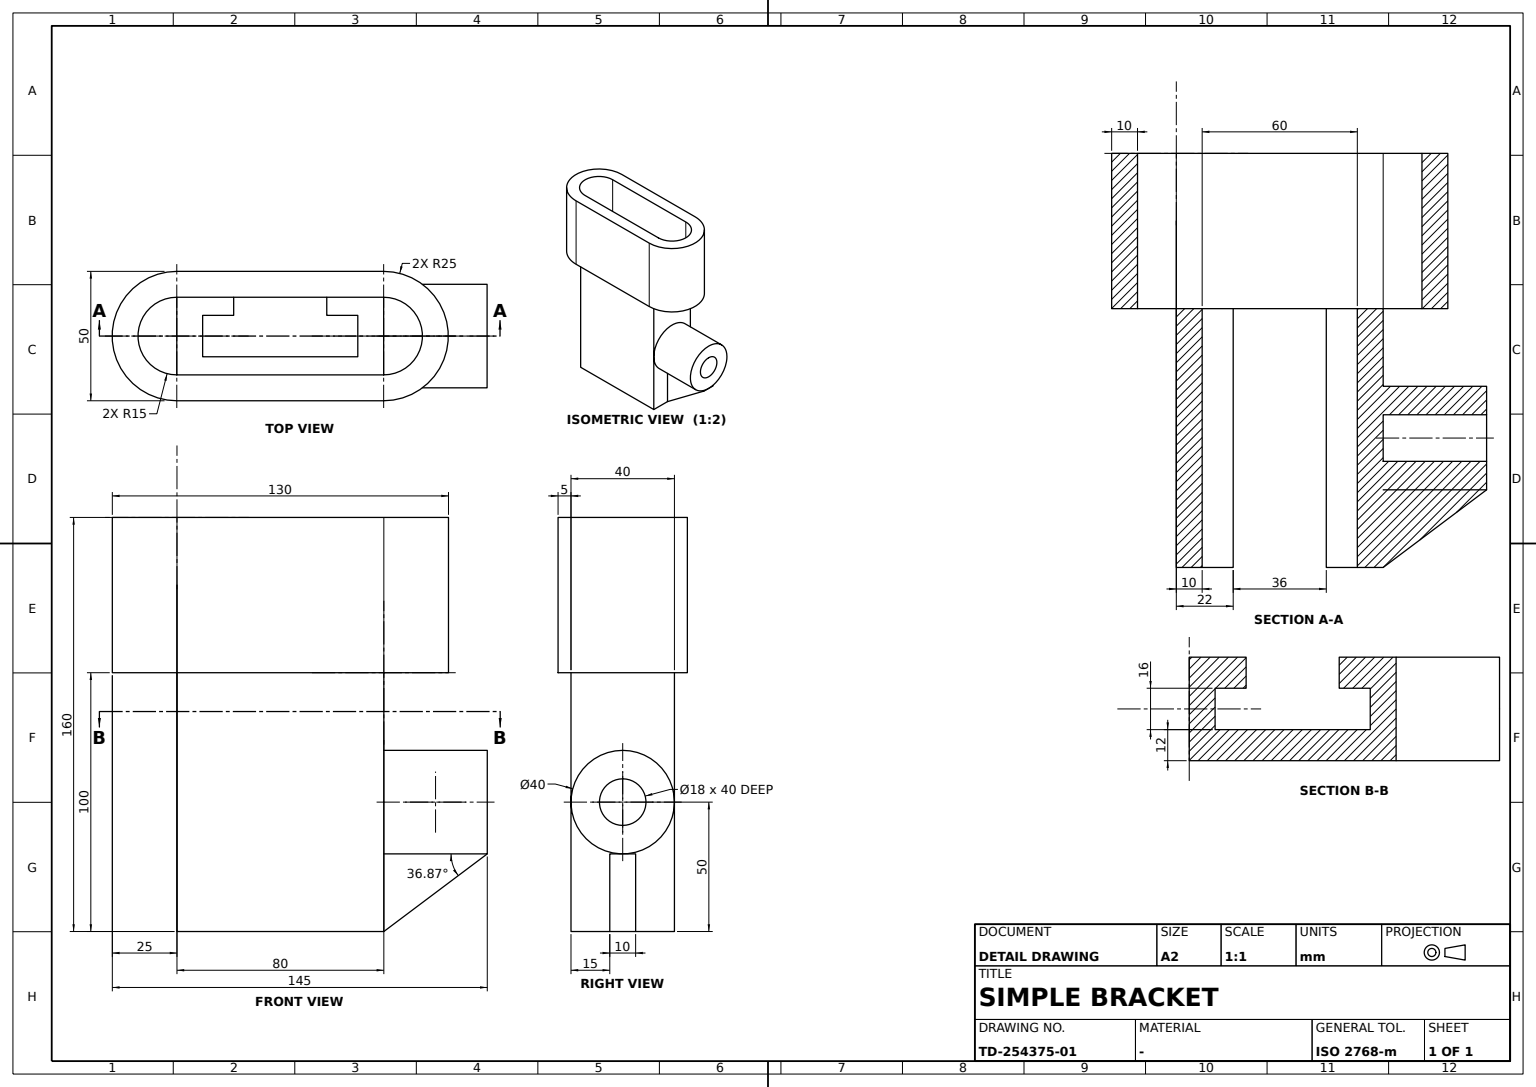
ISO-10303-21;
HEADER;
FILE_DESCRIPTION((''),'2;1');
FILE_NAME('','',(''),(''),'','','');
FILE_SCHEMA(('AUTOMOTIVE_DESIGN'));
ENDSEC;
DATA;
#1=APPLICATION_CONTEXT('');
#2=PRODUCT_CONTEXT('',#1,'mechanical');
#3=PRODUCT('','','',(#2));
#4=PRODUCT_DEFINITION_FORMATION('','',#3);
#5=PRODUCT_DEFINITION_CONTEXT('',#1,'design');
#6=PRODUCT_DEFINITION('','',#4,#5);
#7=PRODUCT_DEFINITION_SHAPE('','',#6);
#8=(LENGTH_UNIT()NAMED_UNIT(*)SI_UNIT(.MILLI.,.METRE.));
#9=(NAMED_UNIT(*)PLANE_ANGLE_UNIT()SI_UNIT($,.RADIAN.));
#10=(NAMED_UNIT(*)SI_UNIT($,.STERADIAN.)SOLID_ANGLE_UNIT());
#11=UNCERTAINTY_MEASURE_WITH_UNIT(LENGTH_MEASURE(0.005),#8,'distance_accuracy_value','');
#12=(GEOMETRIC_REPRESENTATION_CONTEXT(3)GLOBAL_UNCERTAINTY_ASSIGNED_CONTEXT((#11))GLOBAL_UNIT_ASSIGNED_CONTEXT((#8,#9,#10))REPRESENTATION_CONTEXT('',''));
#13=CARTESIAN_POINT('',(-15.,-58.,100.));
#14=VERTEX_POINT('',#13);
#15=CARTESIAN_POINT('',(-15.,-80.,100.));
#16=VERTEX_POINT('',#15);
#17=CARTESIAN_POINT('',(-15.,0.,100.));
#18=DIRECTION('',(0.,-1.,0.));
#19=VECTOR('',#18,1000.);
#20=LINE('',#17,#19);
#21=EDGE_CURVE('',#14,#16,#20,.T.);
#22=ORIENTED_EDGE('',*,*,#21,.F.);
#23=CARTESIAN_POINT('',(-15.,-22.,100.));
#24=VERTEX_POINT('',#23);
#25=EDGE_CURVE('',#24,#14,#20,.T.);
#26=ORIENTED_EDGE('',*,*,#25,.F.);
#27=VERTEX_POINT('',#17);
#28=EDGE_CURVE('',#27,#24,#20,.T.);
#29=ORIENTED_EDGE('',*,*,#28,.F.);
#30=CARTESIAN_POINT('',(-15.,0.,160.));
#31=VERTEX_POINT('',#30);
#32=CARTESIAN_POINT('',(-15.,0.,130.));
#33=DIRECTION('',(0.,0.,1.));
#34=VECTOR('',#33,1000.);
#35=LINE('',#32,#34);
#36=EDGE_CURVE('',#27,#31,#35,.T.);
#37=ORIENTED_EDGE('',*,*,#36,.T.);
#38=CARTESIAN_POINT('',(-15.,-80.,160.));
#39=VERTEX_POINT('',#38);
#40=LINE('',#30,#19);
#41=EDGE_CURVE('',#31,#39,#40,.T.);
#42=ORIENTED_EDGE('',*,*,#41,.T.);
#43=CARTESIAN_POINT('',(-15.,-80.,130.));
#44=LINE('',#43,#34);
#45=EDGE_CURVE('',#16,#39,#44,.T.);
#46=ORIENTED_EDGE('',*,*,#45,.F.);
#47=EDGE_LOOP('',(#22,#26,#29,#37,#42,#46));
#48=FACE_BOUND('',#47,.T.);
#49=DIRECTION('',(-1.,0.,0.));
#50=AXIS2_PLACEMENT_3D('',#17,#49,#18);
#51=PLANE('',#50);
#52=ADVANCED_FACE('',(#48),#51,.F.);
#53=CARTESIAN_POINT('',(15.,-80.,160.));
#54=VERTEX_POINT('',#53);
#55=CARTESIAN_POINT('',(0.,-80.,160.));
#56=DIRECTION('',(1.,0.,0.));
#57=AXIS2_PLACEMENT_3D('',#55,#33,#56);
#58=CIRCLE('',#57,15.);
#59=EDGE_CURVE('',#39,#54,#58,.T.);
#60=ORIENTED_EDGE('',*,*,#59,.T.);
#61=CARTESIAN_POINT('',(15.,-80.,100.));
#62=VERTEX_POINT('',#61);
#63=CARTESIAN_POINT('',(15.,-80.,130.));
#64=LINE('',#63,#34);
#65=EDGE_CURVE('',#62,#54,#64,.T.);
#66=ORIENTED_EDGE('',*,*,#65,.F.);
#67=CARTESIAN_POINT('',(0.,-80.,100.));
#68=AXIS2_PLACEMENT_3D('',#67,#33,#56);
#69=CIRCLE('',#68,15.);
#70=EDGE_CURVE('',#16,#62,#69,.T.);
#71=ORIENTED_EDGE('',*,*,#70,.F.);
#72=ORIENTED_EDGE('',*,*,#45,.T.);
#73=EDGE_LOOP('',(#60,#66,#71,#72));
#74=FACE_BOUND('',#73,.T.);
#75=CARTESIAN_POINT('',(0.,-80.,130.));
#76=AXIS2_PLACEMENT_3D('',#75,#33,#56);
#77=CYLINDRICAL_SURFACE('',#76,15.);
#78=ADVANCED_FACE('',(#74),#77,.F.);
#79=CARTESIAN_POINT('',(-8.,-58.,0.));
#80=VERTEX_POINT('',#79);
#81=CARTESIAN_POINT('',(-8.,-70.,0.));
#82=VERTEX_POINT('',#81);
#83=CARTESIAN_POINT('',(-8.,0.,0.));
#84=LINE('',#83,#19);
#85=EDGE_CURVE('',#80,#82,#84,.T.);
#86=ORIENTED_EDGE('',*,*,#85,.F.);
#87=CARTESIAN_POINT('',(-8.,-58.,100.));
#88=VERTEX_POINT('',#87);
#89=LINE('',#79,#34);
#90=EDGE_CURVE('',#80,#88,#89,.T.);
#91=ORIENTED_EDGE('',*,*,#90,.T.);
#92=CARTESIAN_POINT('',(-8.,-70.,100.));
#93=VERTEX_POINT('',#92);
#94=CARTESIAN_POINT('',(-8.,0.,100.));
#95=LINE('',#94,#19);
#96=EDGE_CURVE('',#88,#93,#95,.T.);
#97=ORIENTED_EDGE('',*,*,#96,.T.);
#98=LINE('',#81,#34);
#99=EDGE_CURVE('',#82,#93,#98,.T.);
#100=ORIENTED_EDGE('',*,*,#99,.F.);
#101=EDGE_LOOP('',(#86,#91,#97,#100));
#102=FACE_BOUND('',#101,.T.);
#103=CARTESIAN_POINT('',(-8.,-10.,0.));
#104=AXIS2_PLACEMENT_3D('',#103,#49,#18);
#105=PLANE('',#104);
#106=ADVANCED_FACE('',(#102),#105,.F.);
#107=CARTESIAN_POINT('',(-20.,-58.,0.));
#108=VERTEX_POINT('',#107);
#109=CARTESIAN_POINT('',(0.,-58.,0.));
#110=VECTOR('',#56,1000.);
#111=LINE('',#109,#110);
#112=EDGE_CURVE('',#108,#80,#111,.T.);
#113=ORIENTED_EDGE('',*,*,#112,.F.);
#114=CARTESIAN_POINT('',(-20.,-58.,100.));
#115=VERTEX_POINT('',#114);
#116=LINE('',#107,#34);
#117=EDGE_CURVE('',#108,#115,#116,.T.);
#118=ORIENTED_EDGE('',*,*,#117,.T.);
#119=CARTESIAN_POINT('',(0.,-58.,100.));
#120=LINE('',#119,#110);
#121=EDGE_CURVE('',#115,#14,#120,.T.);
#122=ORIENTED_EDGE('',*,*,#121,.T.);
#123=EDGE_CURVE('',#14,#88,#120,.T.);
#124=ORIENTED_EDGE('',*,*,#123,.T.);
#125=ORIENTED_EDGE('',*,*,#90,.F.);
#126=EDGE_LOOP('',(#113,#118,#122,#124,#125));
#127=FACE_BOUND('',#126,.T.);
#128=AXIS2_PLACEMENT_3D('',#107,#18,#56);
#129=PLANE('',#128);
#130=ADVANCED_FACE('',(#127),#129,.F.);
#131=CARTESIAN_POINT('',(-5.,0.,0.));
#132=VERTEX_POINT('',#131);
#133=CARTESIAN_POINT('',(-5.,40.,30.));
#134=VERTEX_POINT('',#133);
#135=DIRECTION('',(0.,0.8,0.6));
#136=VECTOR('',#135,1000.);
#137=LINE('',#131,#136);
#138=EDGE_CURVE('',#132,#134,#137,.T.);
#139=ORIENTED_EDGE('',*,*,#138,.F.);
#140=CARTESIAN_POINT('',(-5.,0.,30.));
#141=VERTEX_POINT('',#140);
#142=DIRECTION('',(0.,0.,-1.));
#143=VECTOR('',#142,1000.);
#144=LINE('',#131,#143);
#145=EDGE_CURVE('',#141,#132,#144,.T.);
#146=ORIENTED_EDGE('',*,*,#145,.F.);
#147=LINE('',#140,#19);
#148=EDGE_CURVE('',#134,#141,#147,.T.);
#149=ORIENTED_EDGE('',*,*,#148,.F.);
#150=EDGE_LOOP('',(#139,#146,#149));
#151=FACE_BOUND('',#150,.T.);
#152=DIRECTION('',(0.,1.,0.));
#153=AXIS2_PLACEMENT_3D('',#131,#56,#152);
#154=PLANE('',#153);
#155=ADVANCED_FACE('',(#151),#154,.F.);
#156=ORIENTED_EDGE('',*,*,#148,.T.);
#157=CARTESIAN_POINT('',(0.,0.,30.));
#158=VERTEX_POINT('',#157);
#159=LINE('',#157,#110);
#160=EDGE_CURVE('',#141,#158,#159,.T.);
#161=ORIENTED_EDGE('',*,*,#160,.T.);
#162=CARTESIAN_POINT('',(5.,0.,30.));
#163=VERTEX_POINT('',#162);
#164=EDGE_CURVE('',#158,#163,#159,.T.);
#165=ORIENTED_EDGE('',*,*,#164,.T.);
#166=CARTESIAN_POINT('',(5.,40.,30.));
#167=VERTEX_POINT('',#166);
#168=LINE('',#162,#19);
#169=EDGE_CURVE('',#167,#163,#168,.T.);
#170=ORIENTED_EDGE('',*,*,#169,.F.);
#171=CARTESIAN_POINT('',(0.,40.,30.));
#172=LINE('',#171,#110);
#173=EDGE_CURVE('',#134,#167,#172,.T.);
#174=ORIENTED_EDGE('',*,*,#173,.F.);
#175=EDGE_LOOP('',(#156,#161,#165,#170,#174));
#176=FACE_BOUND('',#175,.T.);
#177=AXIS2_PLACEMENT_3D('',#171,#33,#18);
#178=PLANE('',#177);
#179=ADVANCED_FACE('',(#176),#178,.T.);
#180=CARTESIAN_POINT('',(-8.,-22.,100.));
#181=VERTEX_POINT('',#180);
#182=CARTESIAN_POINT('',(0.,-22.,100.));
#183=VECTOR('',#49,1000.);
#184=LINE('',#182,#183);
#185=EDGE_CURVE('',#181,#24,#184,.T.);
#186=ORIENTED_EDGE('',*,*,#185,.T.);
#187=CARTESIAN_POINT('',(-20.,-22.,100.));
#188=VERTEX_POINT('',#187);
#189=EDGE_CURVE('',#24,#188,#184,.T.);
#190=ORIENTED_EDGE('',*,*,#189,.T.);
#191=CARTESIAN_POINT('',(-20.,-22.,0.));
#192=VERTEX_POINT('',#191);
#193=LINE('',#191,#34);
#194=EDGE_CURVE('',#192,#188,#193,.T.);
#195=ORIENTED_EDGE('',*,*,#194,.F.);
#196=CARTESIAN_POINT('',(-8.,-22.,0.));
#197=VERTEX_POINT('',#196);
#198=CARTESIAN_POINT('',(0.,-22.,0.));
#199=LINE('',#198,#183);
#200=EDGE_CURVE('',#197,#192,#199,.T.);
#201=ORIENTED_EDGE('',*,*,#200,.F.);
#202=LINE('',#196,#34);
#203=EDGE_CURVE('',#197,#181,#202,.T.);
#204=ORIENTED_EDGE('',*,*,#203,.T.);
#205=EDGE_LOOP('',(#186,#190,#195,#201,#204));
#206=FACE_BOUND('',#205,.T.);
#207=AXIS2_PLACEMENT_3D('',#196,#152,#49);
#208=PLANE('',#207);
#209=ADVANCED_FACE('',(#206),#208,.F.);
#210=ORIENTED_EDGE('',*,*,#203,.F.);
#211=VERTEX_POINT('',#103);
#212=EDGE_CURVE('',#211,#197,#84,.T.);
#213=ORIENTED_EDGE('',*,*,#212,.F.);
#214=CARTESIAN_POINT('',(-8.,-10.,100.));
#215=VERTEX_POINT('',#214);
#216=LINE('',#103,#34);
#217=EDGE_CURVE('',#211,#215,#216,.T.);
#218=ORIENTED_EDGE('',*,*,#217,.T.);
#219=EDGE_CURVE('',#215,#181,#95,.T.);
#220=ORIENTED_EDGE('',*,*,#219,.T.);
#221=EDGE_LOOP('',(#210,#213,#218,#220));
#222=FACE_BOUND('',#221,.T.);
#223=ADVANCED_FACE('',(#222),#105,.F.);
#224=ORIENTED_EDGE('',*,*,#112,.T.);
#225=ORIENTED_EDGE('',*,*,#85,.T.);
#226=CARTESIAN_POINT('',(8.,-70.,0.));
#227=VERTEX_POINT('',#226);
#228=CARTESIAN_POINT('',(0.,-70.,0.));
#229=LINE('',#228,#110);
#230=EDGE_CURVE('',#82,#227,#229,.T.);
#231=ORIENTED_EDGE('',*,*,#230,.T.);
#232=CARTESIAN_POINT('',(8.,-10.,0.));
#233=VERTEX_POINT('',#232);
#234=CARTESIAN_POINT('',(8.,0.,0.));
#235=VECTOR('',#152,1000.);
#236=LINE('',#234,#235);
#237=EDGE_CURVE('',#227,#233,#236,.T.);
#238=ORIENTED_EDGE('',*,*,#237,.T.);
#239=CARTESIAN_POINT('',(0.,-10.,0.));
#240=LINE('',#239,#183);
#241=EDGE_CURVE('',#233,#211,#240,.T.);
#242=ORIENTED_EDGE('',*,*,#241,.T.);
#243=ORIENTED_EDGE('',*,*,#212,.T.);
#244=ORIENTED_EDGE('',*,*,#200,.T.);
#245=CARTESIAN_POINT('',(-20.,0.,0.));
#246=VERTEX_POINT('',#245);
#247=LINE('',#245,#235);
#248=EDGE_CURVE('',#192,#246,#247,.T.);
#249=ORIENTED_EDGE('',*,*,#248,.T.);
#250=CARTESIAN_POINT('',(0.,0.,0.));
#251=LINE('',#250,#110);
#252=EDGE_CURVE('',#246,#132,#251,.T.);
#253=ORIENTED_EDGE('',*,*,#252,.T.);
#254=CARTESIAN_POINT('',(5.,0.,0.));
#255=VERTEX_POINT('',#254);
#256=EDGE_CURVE('',#132,#255,#251,.T.);
#257=ORIENTED_EDGE('',*,*,#256,.T.);
#258=CARTESIAN_POINT('',(20.,0.,0.));
#259=VERTEX_POINT('',#258);
#260=EDGE_CURVE('',#255,#259,#251,.T.);
#261=ORIENTED_EDGE('',*,*,#260,.T.);
#262=CARTESIAN_POINT('',(20.,-80.,0.));
#263=VERTEX_POINT('',#262);
#264=LINE('',#258,#19);
#265=EDGE_CURVE('',#259,#263,#264,.T.);
#266=ORIENTED_EDGE('',*,*,#265,.T.);
#267=CARTESIAN_POINT('',(-20.,-80.,0.));
#268=VERTEX_POINT('',#267);
#269=CARTESIAN_POINT('',(0.,-80.,0.));
#270=LINE('',#269,#183);
#271=EDGE_CURVE('',#263,#268,#270,.T.);
#272=ORIENTED_EDGE('',*,*,#271,.T.);
#273=EDGE_CURVE('',#268,#108,#247,.T.);
#274=ORIENTED_EDGE('',*,*,#273,.T.);
#275=EDGE_LOOP('',(#224,#225,#231,#238,#242,#243,#244,#249,#253,#257,#261,#266,#272,#274));
#276=FACE_BOUND('',#275,.T.);
#277=AXIS2_PLACEMENT_3D('',#250,#33,#56);
#278=PLANE('',#277);
#279=ADVANCED_FACE('',(#276),#278,.F.);
#280=ORIENTED_EDGE('',*,*,#194,.T.);
#281=CARTESIAN_POINT('',(-20.,0.,100.));
#282=VERTEX_POINT('',#281);
#283=LINE('',#281,#235);
#284=EDGE_CURVE('',#188,#282,#283,.T.);
#285=ORIENTED_EDGE('',*,*,#284,.T.);
#286=CARTESIAN_POINT('',(-20.,0.,50.));
#287=VERTEX_POINT('',#286);
#288=LINE('',#245,#34);
#289=EDGE_CURVE('',#287,#282,#288,.T.);
#290=ORIENTED_EDGE('',*,*,#289,.F.);
#291=EDGE_CURVE('',#246,#287,#288,.T.);
#292=ORIENTED_EDGE('',*,*,#291,.F.);
#293=ORIENTED_EDGE('',*,*,#248,.F.);
#294=EDGE_LOOP('',(#280,#285,#290,#292,#293));
#295=FACE_BOUND('',#294,.T.);
#296=AXIS2_PLACEMENT_3D('',#191,#56,#152);
#297=PLANE('',#296);
#298=ADVANCED_FACE('',(#295),#297,.F.);
#299=CARTESIAN_POINT('',(25.,0.,100.));
#300=VERTEX_POINT('',#299);
#301=CARTESIAN_POINT('',(-25.,0.,100.));
#302=VERTEX_POINT('',#301);
#303=CARTESIAN_POINT('',(0.,0.,100.));
#304=AXIS2_PLACEMENT_3D('',#303,#33,#56);
#305=CIRCLE('',#304,25.);
#306=EDGE_CURVE('',#300,#302,#305,.T.);
#307=ORIENTED_EDGE('',*,*,#306,.T.);
#308=CARTESIAN_POINT('',(-25.,0.,160.));
#309=VERTEX_POINT('',#308);
#310=CARTESIAN_POINT('',(-25.,0.,130.));
#311=LINE('',#310,#34);
#312=EDGE_CURVE('',#302,#309,#311,.T.);
#313=ORIENTED_EDGE('',*,*,#312,.T.);
#314=CARTESIAN_POINT('',(25.,0.,160.));
#315=VERTEX_POINT('',#314);
#316=CARTESIAN_POINT('',(0.,0.,160.));
#317=AXIS2_PLACEMENT_3D('',#316,#33,#56);
#318=CIRCLE('',#317,25.);
#319=EDGE_CURVE('',#315,#309,#318,.T.);
#320=ORIENTED_EDGE('',*,*,#319,.F.);
#321=CARTESIAN_POINT('',(25.,0.,130.));
#322=LINE('',#321,#34);
#323=EDGE_CURVE('',#300,#315,#322,.T.);
#324=ORIENTED_EDGE('',*,*,#323,.F.);
#325=EDGE_LOOP('',(#307,#313,#320,#324));
#326=FACE_BOUND('',#325,.T.);
#327=CARTESIAN_POINT('',(0.,0.,130.));
#328=AXIS2_PLACEMENT_3D('',#327,#33,#56);
#329=CYLINDRICAL_SURFACE('',#328,25.);
#330=ADVANCED_FACE('',(#326),#329,.T.);
#331=CARTESIAN_POINT('',(25.,-80.,100.));
#332=VERTEX_POINT('',#331);
#333=CARTESIAN_POINT('',(25.,-80.,160.));
#334=VERTEX_POINT('',#333);
#335=CARTESIAN_POINT('',(25.,-80.,130.));
#336=LINE('',#335,#34);
#337=EDGE_CURVE('',#332,#334,#336,.T.);
#338=ORIENTED_EDGE('',*,*,#337,.T.);
#339=CARTESIAN_POINT('',(-25.,-80.,160.));
#340=VERTEX_POINT('',#339);
#341=CIRCLE('',#57,25.);
#342=EDGE_CURVE('',#340,#334,#341,.T.);
#343=ORIENTED_EDGE('',*,*,#342,.F.);
#344=CARTESIAN_POINT('',(-25.,-80.,100.));
#345=VERTEX_POINT('',#344);
#346=CARTESIAN_POINT('',(-25.,-80.,130.));
#347=LINE('',#346,#34);
#348=EDGE_CURVE('',#345,#340,#347,.T.);
#349=ORIENTED_EDGE('',*,*,#348,.F.);
#350=CIRCLE('',#68,25.);
#351=EDGE_CURVE('',#345,#332,#350,.T.);
#352=ORIENTED_EDGE('',*,*,#351,.T.);
#353=EDGE_LOOP('',(#338,#343,#349,#352));
#354=FACE_BOUND('',#353,.T.);
#355=CYLINDRICAL_SURFACE('',#76,25.);
#356=ADVANCED_FACE('',(#354),#355,.T.);
#357=CARTESIAN_POINT('',(0.,0.,41.));
#358=VERTEX_POINT('',#357);
#359=CARTESIAN_POINT('',(0.,0.,50.));
#360=AXIS2_PLACEMENT_3D('',#359,#18,#142);
#361=CIRCLE('',#360,9.);
#362=EDGE_CURVE('',#358,#358,#361,.F.);
#363=ORIENTED_EDGE('',*,*,#362,.T.);
#364=EDGE_LOOP('',(#363));
#365=FACE_BOUND('',#364,.T.);
#366=AXIS2_PLACEMENT_3D('',#245,#18,#56);
#367=PLANE('',#366);
#368=ADVANCED_FACE('',(#365),#367,.F.);
#369=CARTESIAN_POINT('',(15.,0.,100.));
#370=VERTEX_POINT('',#369);
#371=CIRCLE('',#304,15.);
#372=EDGE_CURVE('',#370,#27,#371,.T.);
#373=ORIENTED_EDGE('',*,*,#372,.F.);
#374=CARTESIAN_POINT('',(15.,0.,160.));
#375=VERTEX_POINT('',#374);
#376=CARTESIAN_POINT('',(15.,0.,130.));
#377=LINE('',#376,#34);
#378=EDGE_CURVE('',#370,#375,#377,.T.);
#379=ORIENTED_EDGE('',*,*,#378,.T.);
#380=CIRCLE('',#317,15.);
#381=EDGE_CURVE('',#375,#31,#380,.T.);
#382=ORIENTED_EDGE('',*,*,#381,.T.);
#383=ORIENTED_EDGE('',*,*,#36,.F.);
#384=EDGE_LOOP('',(#373,#379,#382,#383));
#385=FACE_BOUND('',#384,.T.);
#386=CYLINDRICAL_SURFACE('',#328,15.);
#387=ADVANCED_FACE('',(#385),#386,.F.);
#388=CARTESIAN_POINT('',(8.,-10.,100.));
#389=VERTEX_POINT('',#388);
#390=CARTESIAN_POINT('',(0.,-10.,100.));
#391=LINE('',#390,#183);
#392=EDGE_CURVE('',#389,#215,#391,.T.);
#393=ORIENTED_EDGE('',*,*,#392,.T.);
#394=ORIENTED_EDGE('',*,*,#217,.F.);
#395=ORIENTED_EDGE('',*,*,#241,.F.);
#396=LINE('',#232,#34);
#397=EDGE_CURVE('',#233,#389,#396,.T.);
#398=ORIENTED_EDGE('',*,*,#397,.T.);
#399=EDGE_LOOP('',(#393,#394,#395,#398));
#400=FACE_BOUND('',#399,.T.);
#401=AXIS2_PLACEMENT_3D('',#232,#152,#49);
#402=PLANE('',#401);
#403=ADVANCED_FACE('',(#400),#402,.F.);
#404=CIRCLE('',#360,20.);
#405=EDGE_CURVE('',#158,#287,#404,.F.);
#406=ORIENTED_EDGE('',*,*,#405,.T.);
#407=CARTESIAN_POINT('',(20.,0.,50.));
#408=VERTEX_POINT('',#407);
#409=EDGE_CURVE('',#287,#408,#404,.F.);
#410=ORIENTED_EDGE('',*,*,#409,.T.);
#411=EDGE_CURVE('',#408,#158,#404,.F.);
#412=ORIENTED_EDGE('',*,*,#411,.T.);
#413=EDGE_LOOP('',(#406,#410,#412));
#414=FACE_BOUND('',#413,.T.);
#415=CARTESIAN_POINT('',(0.,40.,70.));
#416=VERTEX_POINT('',#415);
#417=CARTESIAN_POINT('',(0.,40.,50.));
#418=AXIS2_PLACEMENT_3D('',#417,#152,#33);
#419=CIRCLE('',#418,20.);
#420=EDGE_CURVE('',#416,#416,#419,.T.);
#421=ORIENTED_EDGE('',*,*,#420,.F.);
#422=EDGE_LOOP('',(#421));
#423=FACE_BOUND('',#422,.T.);
#424=CARTESIAN_POINT('',(0.,20.,50.));
#425=AXIS2_PLACEMENT_3D('',#424,#152,#49);
#426=CYLINDRICAL_SURFACE('',#425,20.);
#427=ADVANCED_FACE('',(#414,#423),#426,.T.);
#428=ORIENTED_EDGE('',*,*,#273,.F.);
#429=CARTESIAN_POINT('',(-20.,-80.,100.));
#430=VERTEX_POINT('',#429);
#431=LINE('',#267,#34);
#432=EDGE_CURVE('',#268,#430,#431,.T.);
#433=ORIENTED_EDGE('',*,*,#432,.T.);
#434=EDGE_CURVE('',#430,#115,#283,.T.);
#435=ORIENTED_EDGE('',*,*,#434,.T.);
#436=ORIENTED_EDGE('',*,*,#117,.F.);
#437=EDGE_LOOP('',(#428,#433,#435,#436));
#438=FACE_BOUND('',#437,.T.);
#439=ADVANCED_FACE('',(#438),#297,.F.);
#440=CARTESIAN_POINT('',(0.,40.,59.));
#441=VERTEX_POINT('',#440);
#442=CIRCLE('',#418,9.);
#443=EDGE_CURVE('',#441,#441,#442,.T.);
#444=ORIENTED_EDGE('',*,*,#443,.F.);
#445=EDGE_LOOP('',(#444));
#446=FACE_BOUND('',#445,.T.);
#447=ORIENTED_EDGE('',*,*,#420,.T.);
#448=EDGE_LOOP('',(#447));
#449=FACE_BOUND('',#448,.T.);
#450=CARTESIAN_POINT('',(0.,40.,0.));
#451=AXIS2_PLACEMENT_3D('',#450,#152,#49);
#452=PLANE('',#451);
#453=ADVANCED_FACE('',(#446,#449),#452,.T.);
#454=LINE('',#254,#136);
#455=EDGE_CURVE('',#255,#167,#454,.T.);
#456=ORIENTED_EDGE('',*,*,#455,.T.);
#457=ORIENTED_EDGE('',*,*,#169,.T.);
#458=LINE('',#254,#143);
#459=EDGE_CURVE('',#163,#255,#458,.T.);
#460=ORIENTED_EDGE('',*,*,#459,.T.);
#461=EDGE_LOOP('',(#456,#457,#460));
#462=FACE_BOUND('',#461,.T.);
#463=AXIS2_PLACEMENT_3D('',#254,#56,#152);
#464=PLANE('',#463);
#465=ADVANCED_FACE('',(#462),#464,.T.);
#466=ORIENTED_EDGE('',*,*,#455,.F.);
#467=ORIENTED_EDGE('',*,*,#256,.F.);
#468=ORIENTED_EDGE('',*,*,#138,.T.);
#469=ORIENTED_EDGE('',*,*,#173,.T.);
#470=EDGE_LOOP('',(#466,#467,#468,#469));
#471=FACE_BOUND('',#470,.T.);
#472=DIRECTION('',(0.,0.6,-0.8));
#473=AXIS2_PLACEMENT_3D('',#250,#472,#135);
#474=PLANE('',#473);
#475=ADVANCED_FACE('',(#471),#474,.T.);
#476=ORIENTED_EDGE('',*,*,#443,.T.);
#477=EDGE_LOOP('',(#476));
#478=FACE_BOUND('',#477,.T.);
#479=ORIENTED_EDGE('',*,*,#362,.F.);
#480=EDGE_LOOP('',(#479));
#481=FACE_BOUND('',#480,.T.);
#482=CYLINDRICAL_SURFACE('',#425,9.);
#483=ADVANCED_FACE('',(#478,#481),#482,.F.);
#484=CARTESIAN_POINT('',(20.,0.,100.));
#485=VERTEX_POINT('',#484);
#486=LINE('',#258,#34);
#487=EDGE_CURVE('',#408,#485,#486,.T.);
#488=ORIENTED_EDGE('',*,*,#487,.T.);
#489=CARTESIAN_POINT('',(20.,-80.,100.));
#490=VERTEX_POINT('',#489);
#491=LINE('',#484,#19);
#492=EDGE_CURVE('',#485,#490,#491,.T.);
#493=ORIENTED_EDGE('',*,*,#492,.T.);
#494=LINE('',#262,#34);
#495=EDGE_CURVE('',#263,#490,#494,.T.);
#496=ORIENTED_EDGE('',*,*,#495,.F.);
#497=ORIENTED_EDGE('',*,*,#265,.F.);
#498=EDGE_CURVE('',#259,#408,#486,.T.);
#499=ORIENTED_EDGE('',*,*,#498,.T.);
#500=EDGE_LOOP('',(#488,#493,#496,#497,#499));
#501=FACE_BOUND('',#500,.T.);
#502=AXIS2_PLACEMENT_3D('',#258,#49,#18);
#503=PLANE('',#502);
#504=ADVANCED_FACE('',(#501),#503,.F.);
#505=LINE('',#308,#19);
#506=EDGE_CURVE('',#309,#340,#505,.T.);
#507=ORIENTED_EDGE('',*,*,#506,.F.);
#508=ORIENTED_EDGE('',*,*,#312,.F.);
#509=LINE('',#301,#19);
#510=EDGE_CURVE('',#302,#345,#509,.T.);
#511=ORIENTED_EDGE('',*,*,#510,.T.);
#512=ORIENTED_EDGE('',*,*,#348,.T.);
#513=EDGE_LOOP('',(#507,#508,#511,#512));
#514=FACE_BOUND('',#513,.T.);
#515=AXIS2_PLACEMENT_3D('',#301,#49,#18);
#516=PLANE('',#515);
#517=ADVANCED_FACE('',(#514),#516,.T.);
#518=ORIENTED_EDGE('',*,*,#487,.F.);
#519=ORIENTED_EDGE('',*,*,#409,.F.);
#520=ORIENTED_EDGE('',*,*,#289,.T.);
#521=LINE('',#303,#110);
#522=EDGE_CURVE('',#282,#27,#521,.T.);
#523=ORIENTED_EDGE('',*,*,#522,.T.);
#524=EDGE_CURVE('',#27,#370,#521,.T.);
#525=ORIENTED_EDGE('',*,*,#524,.T.);
#526=EDGE_CURVE('',#370,#485,#521,.T.);
#527=ORIENTED_EDGE('',*,*,#526,.T.);
#528=EDGE_LOOP('',(#518,#519,#520,#523,#525,#527));
#529=FACE_BOUND('',#528,.T.);
#530=ADVANCED_FACE('',(#529),#367,.F.);
#531=ORIENTED_EDGE('',*,*,#291,.T.);
#532=ORIENTED_EDGE('',*,*,#405,.F.);
#533=ORIENTED_EDGE('',*,*,#160,.F.);
#534=ORIENTED_EDGE('',*,*,#145,.T.);
#535=ORIENTED_EDGE('',*,*,#252,.F.);
#536=EDGE_LOOP('',(#531,#532,#533,#534,#535));
#537=FACE_BOUND('',#536,.T.);
#538=ADVANCED_FACE('',(#537),#367,.F.);
#539=LINE('',#299,#19);
#540=EDGE_CURVE('',#300,#332,#539,.T.);
#541=ORIENTED_EDGE('',*,*,#540,.F.);
#542=ORIENTED_EDGE('',*,*,#323,.T.);
#543=LINE('',#314,#19);
#544=EDGE_CURVE('',#315,#334,#543,.T.);
#545=ORIENTED_EDGE('',*,*,#544,.T.);
#546=ORIENTED_EDGE('',*,*,#337,.F.);
#547=EDGE_LOOP('',(#541,#542,#545,#546));
#548=FACE_BOUND('',#547,.T.);
#549=AXIS2_PLACEMENT_3D('',#299,#49,#18);
#550=PLANE('',#549);
#551=ADVANCED_FACE('',(#548),#550,.F.);
#552=CARTESIAN_POINT('',(8.,-70.,100.));
#553=VERTEX_POINT('',#552);
#554=CARTESIAN_POINT('',(8.,0.,100.));
#555=LINE('',#554,#235);
#556=EDGE_CURVE('',#553,#389,#555,.T.);
#557=ORIENTED_EDGE('',*,*,#556,.T.);
#558=ORIENTED_EDGE('',*,*,#397,.F.);
#559=ORIENTED_EDGE('',*,*,#237,.F.);
#560=LINE('',#226,#34);
#561=EDGE_CURVE('',#227,#553,#560,.T.);
#562=ORIENTED_EDGE('',*,*,#561,.T.);
#563=EDGE_LOOP('',(#557,#558,#559,#562));
#564=FACE_BOUND('',#563,.T.);
#565=AXIS2_PLACEMENT_3D('',#226,#56,#152);
#566=PLANE('',#565);
#567=ADVANCED_FACE('',(#564),#566,.F.);
#568=ORIENTED_EDGE('',*,*,#510,.F.);
#569=ORIENTED_EDGE('',*,*,#306,.F.);
#570=ORIENTED_EDGE('',*,*,#540,.T.);
#571=ORIENTED_EDGE('',*,*,#351,.F.);
#572=EDGE_LOOP('',(#568,#569,#570,#571));
#573=FACE_BOUND('',#572,.T.);
#574=ORIENTED_EDGE('',*,*,#526,.F.);
#575=ORIENTED_EDGE('',*,*,#372,.T.);
#576=ORIENTED_EDGE('',*,*,#522,.F.);
#577=ORIENTED_EDGE('',*,*,#284,.F.);
#578=ORIENTED_EDGE('',*,*,#189,.F.);
#579=ORIENTED_EDGE('',*,*,#25,.T.);
#580=ORIENTED_EDGE('',*,*,#121,.F.);
#581=ORIENTED_EDGE('',*,*,#434,.F.);
#582=LINE('',#67,#183);
#583=EDGE_CURVE('',#16,#430,#582,.T.);
#584=ORIENTED_EDGE('',*,*,#583,.F.);
#585=ORIENTED_EDGE('',*,*,#70,.T.);
#586=EDGE_CURVE('',#490,#62,#582,.T.);
#587=ORIENTED_EDGE('',*,*,#586,.F.);
#588=ORIENTED_EDGE('',*,*,#492,.F.);
#589=EDGE_LOOP('',(#574,#575,#576,#577,#578,#579,#580,#581,#584,#585,#587,#588));
#590=FACE_BOUND('',#589,.T.);
#591=PLANE('',#304);
#592=ADVANCED_FACE('',(#573,#590),#591,.F.);
#593=ORIENTED_EDGE('',*,*,#432,.F.);
#594=ORIENTED_EDGE('',*,*,#271,.F.);
#595=ORIENTED_EDGE('',*,*,#495,.T.);
#596=ORIENTED_EDGE('',*,*,#586,.T.);
#597=EDGE_CURVE('',#62,#16,#582,.T.);
#598=ORIENTED_EDGE('',*,*,#597,.T.);
#599=ORIENTED_EDGE('',*,*,#583,.T.);
#600=EDGE_LOOP('',(#593,#594,#595,#596,#598,#599));
#601=FACE_BOUND('',#600,.T.);
#602=AXIS2_PLACEMENT_3D('',#262,#152,#49);
#603=PLANE('',#602);
#604=ADVANCED_FACE('',(#601),#603,.F.);
#605=ORIENTED_EDGE('',*,*,#392,.F.);
#606=ORIENTED_EDGE('',*,*,#556,.F.);
#607=CARTESIAN_POINT('',(0.,-70.,100.));
#608=LINE('',#607,#110);
#609=EDGE_CURVE('',#93,#553,#608,.T.);
#610=ORIENTED_EDGE('',*,*,#609,.F.);
#611=ORIENTED_EDGE('',*,*,#96,.F.);
#612=ORIENTED_EDGE('',*,*,#123,.F.);
#613=ORIENTED_EDGE('',*,*,#21,.T.);
#614=ORIENTED_EDGE('',*,*,#597,.F.);
#615=LINE('',#369,#19);
#616=EDGE_CURVE('',#370,#62,#615,.T.);
#617=ORIENTED_EDGE('',*,*,#616,.F.);
#618=ORIENTED_EDGE('',*,*,#524,.F.);
#619=ORIENTED_EDGE('',*,*,#28,.T.);
#620=ORIENTED_EDGE('',*,*,#185,.F.);
#621=ORIENTED_EDGE('',*,*,#219,.F.);
#622=EDGE_LOOP('',(#605,#606,#610,#611,#612,#613,#614,#617,#618,#619,#620,#621));
#623=FACE_BOUND('',#622,.T.);
#624=ADVANCED_FACE('',(#623),#591,.T.);
#625=ORIENTED_EDGE('',*,*,#164,.F.);
#626=ORIENTED_EDGE('',*,*,#411,.F.);
#627=ORIENTED_EDGE('',*,*,#498,.F.);
#628=ORIENTED_EDGE('',*,*,#260,.F.);
#629=ORIENTED_EDGE('',*,*,#459,.F.);
#630=EDGE_LOOP('',(#625,#626,#627,#628,#629));
#631=FACE_BOUND('',#630,.T.);
#632=ADVANCED_FACE('',(#631),#367,.F.);
#633=ORIENTED_EDGE('',*,*,#342,.T.);
#634=ORIENTED_EDGE('',*,*,#544,.F.);
#635=ORIENTED_EDGE('',*,*,#319,.T.);
#636=ORIENTED_EDGE('',*,*,#506,.T.);
#637=EDGE_LOOP('',(#633,#634,#635,#636));
#638=FACE_BOUND('',#637,.T.);
#639=ORIENTED_EDGE('',*,*,#41,.F.);
#640=ORIENTED_EDGE('',*,*,#381,.F.);
#641=LINE('',#374,#19);
#642=EDGE_CURVE('',#375,#54,#641,.T.);
#643=ORIENTED_EDGE('',*,*,#642,.T.);
#644=ORIENTED_EDGE('',*,*,#59,.F.);
#645=EDGE_LOOP('',(#639,#640,#643,#644));
#646=FACE_BOUND('',#645,.T.);
#647=PLANE('',#317);
#648=ADVANCED_FACE('',(#638,#646),#647,.T.);
#649=ORIENTED_EDGE('',*,*,#616,.T.);
#650=ORIENTED_EDGE('',*,*,#65,.T.);
#651=ORIENTED_EDGE('',*,*,#642,.F.);
#652=ORIENTED_EDGE('',*,*,#378,.F.);
#653=EDGE_LOOP('',(#649,#650,#651,#652));
#654=FACE_BOUND('',#653,.T.);
#655=AXIS2_PLACEMENT_3D('',#369,#49,#18);
#656=PLANE('',#655);
#657=ADVANCED_FACE('',(#654),#656,.T.);
#658=ORIENTED_EDGE('',*,*,#561,.F.);
#659=ORIENTED_EDGE('',*,*,#230,.F.);
#660=ORIENTED_EDGE('',*,*,#99,.T.);
#661=ORIENTED_EDGE('',*,*,#609,.T.);
#662=EDGE_LOOP('',(#658,#659,#660,#661));
#663=FACE_BOUND('',#662,.T.);
#664=AXIS2_PLACEMENT_3D('',#81,#18,#56);
#665=PLANE('',#664);
#666=ADVANCED_FACE('',(#663),#665,.F.);
#667=CLOSED_SHELL('',(#52,#78,#106,#130,#155,#179,#209,#223,#279,#298,#330,#356,#368,#387,#403,#427,#439,#453,#465,#475,#483,#504,#517,#530,#538,#551,#567,#592,#604,#624,#632,#648,#657,#666));
#668=MANIFOLD_SOLID_BREP('',#667);
#669=ADVANCED_BREP_SHAPE_REPRESENTATION('',(#668),#12);
#670=SHAPE_DEFINITION_REPRESENTATION(#7,#669);
ENDSEC;
END-ISO-10303-21;
